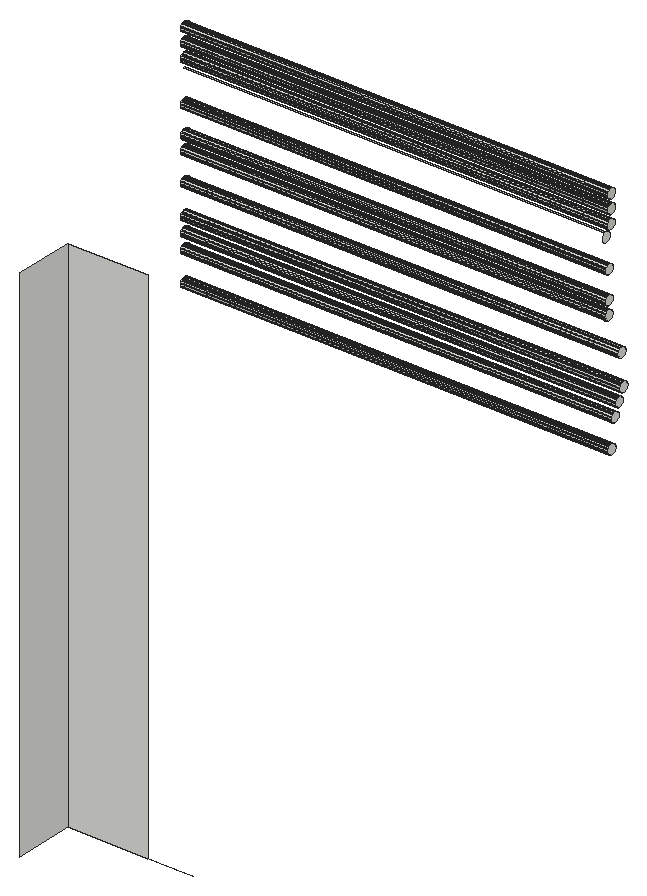
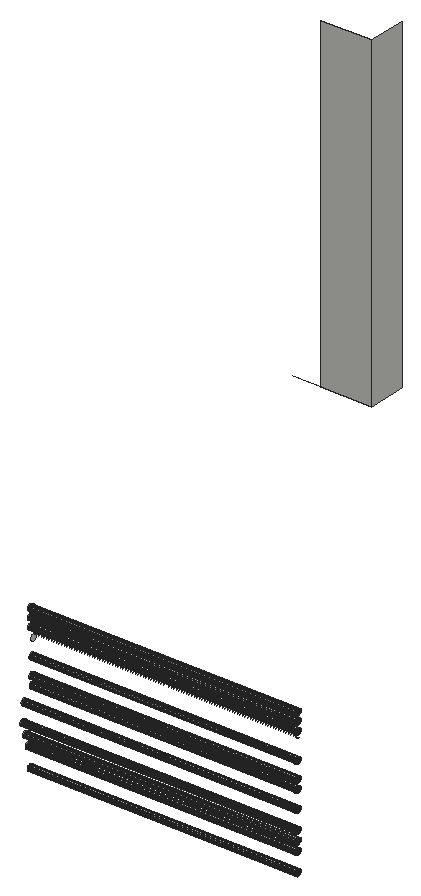
# SketchUp Ruby script. Lengths in inches.
U = 1.inch
M = Sketchup.active_model
def pt(a) = Geom::Point3d.new(a.map { |v| v * U })
def face(e, loops, mat)
  f = e.add_face(loops[0].map { |a| pt(a) })
  loops[1..].each { |l| e.add_face(l.map { |a| pt(a) }).erase! }
  f.material = f.back_material = mat if mat
  f
end
# faces: each face lists its corners as indices into pts; further lists are holes
def faces(e, pts, list, mat = nil) = list.each { |f| face(e, (f[0].is_a?(Array) ? f : [f]).map { |l| l.map { |i| pts[i] } }, mat) }
# xy, xz, yz: faces in a plane at the given z, y or x. An outline is a flat list of corners, or four numbers for a rectangle; further outlines are holes
def ring(l) = l.size == 4 ? [[l[0], l[1]], [l[2], l[1]], [l[2], l[3]], [l[0], l[3]]] : l.each_slice(2).to_a
def flat(e, list, mat, &to3) = list.each { |f| face(e, (f[0].is_a?(Array) ? f : [f]).map { |l| ring(l).map { |u, v| to3.(u, v) } }, mat) }
def xy(e, z, list, mat = nil) = flat(e, list, mat) { |x, y| [x, y, z] }
def xz(e, y, list, mat = nil) = flat(e, list, mat) { |x, z| [x, y, z] }
def yz(e, x, list, mat = nil) = flat(e, list, mat) { |y, z| [x, y, z] }
def lines(e, pts, list) = list.each { |a, b| e.add_line(pt(pts[a]), pt(pts[b])) }
# prism: a flat outline (further loops are holes) pulled along v
def prism(e, loops, v, mat = nil)
  f = face(e, loops, mat); d = Geom::Vector3d.new(v.map { |x| x * U })
  f.pushpull(f.normal.samedirection?(d) ? d.length : -d.length)
end
def box(e, o, s, mat = nil) = prism(e, [[o, [o[0] + s[0], o[1], o[2]], [o[0] + s[0], o[1] + s[1], o[2]], [o[0], o[1] + s[1], o[2]]]], [0, 0, s[2]], mat)
def at(x, y, z, deg = 0) = Geom::Transformation.translation(pt([x, y, z])) * Geom::Transformation.rotation(ORIGIN, Z_AXIS, deg.degrees)
def axes(o, x, y, z) = Geom::Transformation.new([*x, 0, *y, 0, *z, 0, *pt(o).to_a, 1])
def part(name) = M.definitions.add(name)
# library, detail: a bought-in or finely detailed component or shape, given as its bounding box
def library(name, o, s) = part(name).tap { |d| box(d.entities, o, s) }
def detail(e, o, s) = box(e.add_group.entities, o, s)
def put(e, d, t, mat = nil) = e.add_instance(d, t).tap { |i| i.material = mat if mat }
def group(e, t, mat = nil) = e.add_group.tap { |g| g.transformation = t; g.material = mat if mat }.entities
root = M.entities
M.materials.add("[Terrazzo Tile Light]").color = [219, 217, 210]
xz(root,74.42,[[587.04,144,603,248.36]])
yz(root,557.42,[[245.69,162.95,245.94,162.98,246.16,163.08,246.36,163.23,246.5,163.42,246.6,163.65,246.63,163.89,246.6,164.13,246.5,164.36,246.36,164.55,246.16,164.7,245.94,164.79,245.69,164.83,245.45,164.79,245.22,164.7,245.03,164.55,244.88,164.36,244.79,164.13,244.75,163.89,244.79,163.65,244.88,163.42,245.03,163.23,245.22,163.08,245.45,162.98]])
yz(root,557.98,[[245.69,149.2,245.94,149.23,246.16,149.33,246.36,149.48,246.5,149.67,246.6,149.9,246.63,150.14,246.6,150.38,246.5,150.61,246.36,150.8,246.16,150.95,245.94,151.04,245.69,151.08,245.45,151.04,245.22,150.95,245.03,150.8,244.88,150.61,244.79,150.38,244.75,150.14,244.79,149.9,244.88,149.67,245.03,149.48,245.22,149.33,245.45,149.23]])
yz(root,558.04,[[245.69,151.95,245.94,151.98,246.16,152.08,246.36,152.23,246.5,152.42,246.6,152.65,246.63,152.89,246.6,153.13,246.5,153.36,246.36,153.55,246.16,153.7,245.94,153.79,245.69,153.83,245.45,153.79,245.22,153.7,245.03,153.55,244.88,153.36,244.79,153.13,244.75,152.89,244.79,152.65,244.88,152.42,245.03,152.23,245.22,152.08,245.45,151.98],[245.69,157.45,245.94,157.48,246.16,157.58,246.36,157.73,246.5,157.92,246.6,158.15,246.63,158.39,246.6,158.63,246.5,158.86,246.36,159.05,246.16,159.2,245.94,159.29,245.69,159.33,245.45,159.29,245.22,159.2,245.03,159.05,244.88,158.86,244.79,158.63,244.75,158.39,244.79,158.15,244.88,157.92,245.03,157.73,245.22,157.58,245.45,157.48]])
yz(root,558.42,[[245.69,165.7,245.94,165.73,246.16,165.83,246.36,165.98,246.5,166.17,246.6,166.4,246.63,166.64,246.6,166.88,246.5,167.11,246.36,167.3,246.16,167.45,245.94,167.54,245.69,167.58,245.45,167.54,245.22,167.45,245.03,167.3,244.88,167.11,244.79,166.88,244.75,166.64,244.79,166.4,244.88,166.17,245.03,165.98,245.22,165.83,245.45,165.73]],"[Terrazzo Tile Light]")
yz(root,558.48,[[245.69,168.45,245.94,168.48,246.16,168.58,246.36,168.73,246.5,168.92,246.6,169.15,246.63,169.39,246.6,169.63,246.5,169.86,246.36,170.05,246.16,170.2,245.94,170.29,245.69,170.33,245.45,170.29,245.22,170.2,245.03,170.05,244.88,169.86,244.79,169.63,244.75,169.39,244.79,169.15,244.88,168.92,245.03,168.73,245.22,168.58,245.45,168.48],[245.69,171.2,245.94,171.23,246.16,171.33,246.36,171.48,246.5,171.67,246.6,171.9,246.63,172.14,246.6,172.38,246.5,172.61,246.36,172.8,246.16,172.95,245.94,173.04,245.69,173.08,245.45,173.04,245.22,172.95,245.03,172.8,244.88,172.61,244.79,172.38,244.75,172.14,244.79,171.9,244.88,171.67,245.03,171.48,245.22,171.33,245.45,171.23]],"[Terrazzo Tile Light]")
yz(root,558.54,[[245.69,125.45,245.94,125.48,246.16,125.58,246.36,125.73,246.5,125.92,246.6,126.15,246.63,126.39,246.6,126.63,246.5,126.86,246.36,127.05,246.16,127.2,245.94,127.29,245.69,127.33,245.45,127.29,245.22,127.2,245.03,127.05,244.88,126.86,244.79,126.63,244.75,126.39,244.79,126.15,244.88,125.92,245.03,125.73,245.22,125.58,245.45,125.48]])
yz(root,559.23,[[245.69,131.45,245.94,131.48,246.16,131.58,246.36,131.73,246.5,131.92,246.6,132.15,246.63,132.39,246.6,132.63,246.5,132.86,246.36,133.05,246.16,133.2,245.94,133.29,245.69,133.33,245.45,133.29,245.22,133.2,245.03,133.05,244.88,132.86,244.79,132.63,244.75,132.39,244.79,132.15,244.88,131.92,245.03,131.73,245.22,131.58,245.45,131.48]])
yz(root,560.04,[[245.69,134.45,245.94,134.48,246.16,134.58,246.36,134.73,246.5,134.92,246.6,135.15,246.63,135.39,246.6,135.63,246.5,135.86,246.36,136.05,246.16,136.2,245.94,136.29,245.69,136.33,245.45,136.29,245.22,136.2,245.03,136.05,244.88,135.86,244.79,135.63,244.75,135.39,244.79,135.15,244.88,134.92,245.03,134.73,245.22,134.58,245.45,134.48]])
yz(root,560.54,[[245.69,143.45,245.94,143.48,246.16,143.58,246.36,143.73,246.5,143.92,246.6,144.15,246.63,144.39,246.6,144.63,246.5,144.86,246.36,145.05,246.16,145.2,245.94,145.29,245.69,145.33,245.45,145.29,245.22,145.2,245.03,145.05,244.88,144.86,244.79,144.63,244.75,144.39,244.79,144.15,244.88,143.92,245.03,143.73,245.22,143.58,245.45,143.48]])
yz(root,560.92,[[245.69,137.45,245.94,137.48,246.16,137.58,246.36,137.73,246.5,137.92,246.6,138.15,246.63,138.39,246.6,138.63,246.5,138.86,246.36,139.05,246.16,139.2,245.94,139.29,245.69,139.33,245.45,139.29,245.22,139.2,245.03,139.05,244.88,138.86,244.79,138.63,244.75,138.39,244.79,138.15,244.88,137.92,245.03,137.73,245.22,137.58,245.45,137.48]])
yz(root,587.04,[[62.42,144,74.42,248.36]])
p = [[473.23,245.22,125.58],[473.23,245.45,125.48],[558.54,245.45,125.48],[558.54,245.22,125.58],[473.23,245.69,125.45],[558.54,245.69,125.45],
  [473.23,245.94,125.48],[558.54,245.94,125.48],[473.23,246.16,125.58],[558.54,246.16,125.58],[473.23,245.03,125.73],[558.54,245.03,125.73],
  [473.23,246.36,125.73],[558.54,246.36,125.73],[473.23,244.88,125.92],[558.54,244.88,125.92],[473.23,246.5,125.92],[558.54,246.5,125.92],
  [473.23,244.79,126.15],[558.54,244.79,126.15],[473.23,246.6,126.15],[558.54,246.6,126.15],[473.23,244.75,126.39],[558.54,244.75,126.39],
  [473.23,246.63,126.39],[558.54,246.63,126.39],[473.23,244.79,126.63],[558.54,244.79,126.63],[473.23,246.6,126.63],[558.54,246.6,126.63],
  [473.23,244.88,126.86],[558.54,244.88,126.86],[473.23,246.5,126.86],[558.54,246.5,126.86],[473.23,245.03,127.05],[558.54,245.03,127.05],
  [473.23,246.36,127.05],[558.54,246.36,127.05],[473.23,245.22,127.2],[558.54,245.22,127.2],[473.23,246.16,127.2],[558.54,246.16,127.2],
  [473.23,245.45,127.29],[558.54,245.45,127.29],[473.23,245.94,127.29],[558.54,245.94,127.29],[473.23,245.69,127.33],[558.54,245.69,127.33],
  [473.23,245.22,131.58],[473.23,245.45,131.48],[559.23,245.45,131.48],[559.23,245.22,131.58],[473.23,245.69,131.45],[559.23,245.69,131.45],
  [473.23,245.94,131.48],[559.23,245.94,131.48],[473.23,246.16,131.58],[559.23,246.16,131.58],[473.23,245.03,131.73],[559.23,245.03,131.73],
  [473.23,246.36,131.73],[559.23,246.36,131.73],[473.23,244.88,131.92],[559.23,244.88,131.92],[473.23,246.5,131.92],[559.23,246.5,131.92],
  [473.23,244.79,132.15],[559.23,244.79,132.15],[473.23,246.6,132.15],[559.23,246.6,132.15],[473.23,244.75,132.39],[559.23,244.75,132.39],
  [473.23,246.63,132.39],[559.23,246.63,132.39],[473.23,244.79,132.63],[559.23,244.79,132.63],[473.23,246.6,132.63],[559.23,246.6,132.63],
  [473.23,244.88,132.86],[559.23,244.88,132.86],[473.23,246.5,132.86],[559.23,246.5,132.86],[473.23,245.03,133.05],[559.23,245.03,133.05],
  [473.23,246.36,133.05],[559.23,246.36,133.05],[473.23,245.22,133.2],[559.23,245.22,133.2],[473.23,246.16,133.2],[559.23,246.16,133.2],
  [473.23,245.45,133.29],[559.23,245.45,133.29],[473.23,245.94,133.29],[559.23,245.94,133.29],[473.23,245.69,133.33],[559.23,245.69,133.33],
  [473.23,245.22,134.58],[473.23,245.45,134.48],[560.04,245.45,134.48],[560.04,245.22,134.58],[473.23,245.69,134.45],[560.04,245.69,134.45],
  [473.23,245.94,134.48],[560.04,245.94,134.48],[473.23,246.16,134.58],[560.04,246.16,134.58],[473.23,245.03,134.73],[560.04,245.03,134.73],
  [473.23,246.36,134.73],[560.04,246.36,134.73],[473.23,244.88,134.92],[560.04,244.88,134.92],[473.23,246.5,134.92],[560.04,246.5,134.92],
  [473.23,244.79,135.15],[560.04,244.79,135.15],[473.23,246.6,135.15],[560.04,246.6,135.15],[473.23,244.75,135.39],[560.04,244.75,135.39],
  [473.23,246.63,135.39],[560.04,246.63,135.39],[473.23,244.79,135.63],[560.04,244.79,135.63],[473.23,246.6,135.63],[560.04,246.6,135.63],
  [473.23,244.88,135.86],[560.04,244.88,135.86],[473.23,246.5,135.86],[560.04,246.5,135.86],[473.23,245.03,136.05],[560.04,245.03,136.05],
  [473.23,246.36,136.05],[560.04,246.36,136.05],[473.23,245.22,136.2],[560.04,245.22,136.2],[473.23,246.16,136.2],[560.04,246.16,136.2],
  [473.23,245.45,136.29],[560.04,245.45,136.29],[473.23,245.94,136.29],[560.04,245.94,136.29],[473.23,245.69,136.33],[560.04,245.69,136.33],
  [473.23,245.22,137.58],[473.23,245.45,137.48],[560.92,245.45,137.48],[560.92,245.22,137.58],[473.23,245.69,137.45],[560.92,245.69,137.45],
  [473.23,245.94,137.48],[560.92,245.94,137.48],[473.23,246.16,137.58],[560.92,246.16,137.58],[473.23,245.03,137.73],[560.92,245.03,137.73],
  [473.23,246.36,137.73],[560.92,246.36,137.73],[473.23,244.88,137.92],[560.92,244.88,137.92],[473.23,246.5,137.92],[560.92,246.5,137.92],
  [473.23,244.79,138.15],[560.92,244.79,138.15],[473.23,246.6,138.15],[560.92,246.6,138.15],[473.23,244.75,138.39],[560.92,244.75,138.39],
  [473.23,246.63,138.39],[560.92,246.63,138.39],[473.23,244.79,138.63],[560.92,244.79,138.63],[473.23,246.6,138.63],[560.92,246.6,138.63],
  [473.23,244.88,138.86],[560.92,244.88,138.86],[473.23,246.5,138.86],[560.92,246.5,138.86],[473.23,245.03,139.05],[560.92,245.03,139.05],
  [473.23,246.36,139.05],[560.92,246.36,139.05],[473.23,245.22,139.2],[560.92,245.22,139.2],[473.23,246.16,139.2],[560.92,246.16,139.2],
  [473.23,245.45,139.29],[560.92,245.45,139.29],[473.23,245.94,139.29],[560.92,245.94,139.29],[473.23,245.69,139.33],[560.92,245.69,139.33],
  [473.23,245.22,143.58],[473.23,245.45,143.48],[560.54,245.45,143.48],[560.54,245.22,143.58],[473.23,245.69,143.45],[560.54,245.69,143.45],
  [473.23,245.94,143.48],[560.54,245.94,143.48],[473.23,246.16,143.58],[560.54,246.16,143.58],[473.23,245.03,143.73],[560.54,245.03,143.73],
  [473.23,246.36,143.73],[560.54,246.36,143.73],[473.23,244.88,143.92],[560.54,244.88,143.92],[473.23,246.5,143.92],[560.54,246.5,143.92],
  [473.23,244.79,144.15],[560.54,244.79,144.15],[473.23,246.6,144.15],[560.54,246.6,144.15],[473.23,244.75,144.39],[560.54,244.75,144.39],
  [473.23,246.63,144.39],[560.54,246.63,144.39],[473.23,244.79,144.63],[560.54,244.79,144.63],[473.23,246.6,144.63],[560.54,246.6,144.63],
  [473.23,244.88,144.86],[560.54,244.88,144.86],[473.23,246.5,144.86],[560.54,246.5,144.86],[473.23,245.03,145.05],[560.54,245.03,145.05],
  [473.23,246.36,145.05],[560.54,246.36,145.05],[473.23,245.22,145.2],[560.54,245.22,145.2],[473.23,246.16,145.2],[560.54,246.16,145.2],
  [473.23,245.45,145.29],[560.54,245.45,145.29],[473.23,245.94,145.29],[560.54,245.94,145.29],[473.23,245.69,145.33],[560.54,245.69,145.33],
  [473.23,245.22,149.33],[473.23,245.45,149.23],[557.98,245.45,149.23],[557.98,245.22,149.33],[473.23,245.69,149.2],[557.98,245.69,149.2],
  [473.23,245.94,149.23],[557.98,245.94,149.23],[473.23,246.16,149.33],[557.98,246.16,149.33],[473.23,245.03,149.48],[557.98,245.03,149.48],
  [473.23,246.36,149.48],[557.98,246.36,149.48],[473.23,244.88,149.67],[557.98,244.88,149.67],[473.23,246.5,149.67],[557.98,246.5,149.67],
  [473.23,244.79,149.9],[557.98,244.79,149.9],[473.23,246.6,149.9],[557.98,246.6,149.9],[473.23,244.75,150.14],[557.98,244.75,150.14],
  [473.23,246.63,150.14],[557.98,246.63,150.14],[473.23,244.79,150.38],[557.98,244.79,150.38],[473.23,246.6,150.38],[557.98,246.6,150.38],
  [473.23,244.88,150.61],[557.98,244.88,150.61],[473.23,246.5,150.61],[557.98,246.5,150.61],[473.23,245.03,150.8],[557.98,245.03,150.8],
  [473.23,246.36,150.8],[557.98,246.36,150.8],[473.23,245.22,150.95],[557.98,245.22,150.95],[473.23,246.16,150.95],[557.98,246.16,150.95],
  [473.23,245.45,151.04],[557.98,245.45,151.04],[473.23,245.69,151.08],[557.98,245.69,151.08],[473.23,245.94,151.04],[557.98,245.94,151.04],
  [473.23,245.22,152.08],[473.23,245.45,151.98],[558.04,245.45,151.98],[558.04,245.22,152.08],[473.23,245.69,151.95],[558.04,245.69,151.95],
  [473.23,245.94,151.98],[558.04,245.94,151.98],[473.23,246.16,152.08],[558.04,246.16,152.08],[473.23,245.03,152.23],[558.04,245.03,152.23],
  [473.23,246.36,152.23],[558.04,246.36,152.23],[473.23,244.88,152.42],[558.04,244.88,152.42],[473.23,246.5,152.42],[558.04,246.5,152.42],
  [473.23,244.79,152.65],[558.04,244.79,152.65],[473.23,246.6,152.65],[558.04,246.6,152.65],[473.23,244.75,152.89],[558.04,244.75,152.89],
  [473.23,246.63,152.89],[558.04,246.63,152.89],[473.23,244.79,153.13],[558.04,244.79,153.13],[473.23,246.6,153.13],[558.04,246.6,153.13],
  [473.23,244.88,153.36],[558.04,244.88,153.36],[473.23,246.5,153.36],[558.04,246.5,153.36],[473.23,245.03,153.55],[558.04,245.03,153.55],
  [473.23,246.36,153.55],[558.04,246.36,153.55],[473.23,245.22,153.7],[558.04,245.22,153.7],[473.23,246.16,153.7],[558.04,246.16,153.7],
  [473.23,245.45,153.79],[558.04,245.45,153.79],[473.23,245.94,153.79],[558.04,245.94,153.79],[473.23,245.69,153.83],[558.04,245.69,153.83],
  [473.23,245.22,157.58],[473.23,245.45,157.48],[558.04,245.45,157.48],[558.04,245.22,157.58],[473.23,245.69,157.45],[558.04,245.69,157.45],
  [473.23,245.94,157.48],[558.04,245.94,157.48],[473.23,246.16,157.58],[558.04,246.16,157.58],[473.23,245.03,157.73],[558.04,245.03,157.73],
  [473.23,246.36,157.73],[558.04,246.36,157.73],[473.23,244.88,157.92],[558.04,244.88,157.92],[473.23,246.5,157.92],[558.04,246.5,157.92],
  [473.23,244.79,158.15],[558.04,244.79,158.15],[473.23,246.6,158.15],[558.04,246.6,158.15],[473.23,244.75,158.39],[558.04,244.75,158.39],
  [473.23,246.63,158.39],[558.04,246.63,158.39],[473.23,244.79,158.63],[558.04,244.79,158.63],[473.23,246.6,158.63],[558.04,246.6,158.63],
  [473.23,244.88,158.86],[558.04,244.88,158.86],[473.23,246.5,158.86],[558.04,246.5,158.86],[473.23,245.03,159.05],[558.04,245.03,159.05],
  [473.23,246.36,159.05],[558.04,246.36,159.05],[473.23,245.22,159.2],[558.04,245.22,159.2],[473.23,246.16,159.2],[558.04,246.16,159.2],
  [473.23,245.45,159.29],[558.04,245.45,159.29],[473.23,245.94,159.29],[558.04,245.94,159.29],[473.23,245.69,159.33],[558.04,245.69,159.33],
  [473.23,245.69,164.83],[473.23,245.45,164.79],[557.42,245.45,164.79],[557.42,245.69,164.83],[473.23,245.22,165.83],[473.23,245.45,165.73],
  [558.42,245.45,165.73],[558.42,245.22,165.83],[473.23,245.69,165.7],[558.42,245.69,165.7],[473.23,245.94,165.73],[558.42,245.94,165.73],
  [473.23,246.16,165.83],[558.42,246.16,165.83],[473.23,245.03,165.98],[558.42,245.03,165.98],[473.23,246.36,165.98],[558.42,246.36,165.98],
  [473.23,244.88,166.17],[558.42,244.88,166.17],[473.23,246.5,166.17],[558.42,246.5,166.17],[473.23,244.79,166.4],[558.42,244.79,166.4],
  [473.23,246.6,166.4],[558.42,246.6,166.4],[473.23,244.75,166.64],[558.42,244.75,166.64],[473.23,246.63,166.64],[558.42,246.63,166.64],
  [473.23,244.79,166.88],[558.42,244.79,166.88],[473.23,246.6,166.88],[558.42,246.6,166.88],[473.23,244.88,167.11],[558.42,244.88,167.11],
  [473.23,246.5,167.11],[558.42,246.5,167.11],[473.23,245.03,167.3],[558.42,245.03,167.3],[473.23,246.36,167.3],[558.42,246.36,167.3],
  [473.23,245.22,167.45],[558.42,245.22,167.45],[473.23,246.16,167.45],[558.42,246.16,167.45],[473.23,245.45,167.54],[558.42,245.45,167.54],
  [473.23,245.69,167.58],[558.42,245.69,167.58],[473.23,245.94,167.54],[558.42,245.94,167.54],[473.23,245.22,168.58],[473.23,245.45,168.48],
  [558.48,245.45,168.48],[558.48,245.22,168.58],[473.23,245.69,168.45],[558.48,245.69,168.45],[473.23,245.94,168.48],[558.48,245.94,168.48],
  [473.23,246.16,168.58],[558.48,246.16,168.58],[473.23,245.03,168.73],[558.48,245.03,168.73],[473.23,246.36,168.73],[558.48,246.36,168.73],
  [473.23,244.88,168.92],[558.48,244.88,168.92],[473.23,246.5,168.92],[558.48,246.5,168.92],[473.23,244.79,169.15],[558.48,244.79,169.15],
  [473.23,246.6,169.15],[558.48,246.6,169.15],[473.23,244.75,169.39],[558.48,244.75,169.39],[473.23,246.63,169.39],[558.48,246.63,169.39],
  [473.23,244.79,169.63],[558.48,244.79,169.63],[473.23,246.6,169.63],[558.48,246.6,169.63],[473.23,244.88,169.86],[558.48,244.88,169.86],
  [473.23,246.5,169.86],[558.48,246.5,169.86],[473.23,245.03,170.05],[558.48,245.03,170.05],[473.23,246.36,170.05],[558.48,246.36,170.05],
  [473.23,245.22,170.2],[558.48,245.22,170.2],[473.23,246.16,170.2],[558.48,246.16,170.2],[473.23,245.45,170.29],[558.48,245.45,170.29],
  [473.23,245.94,170.29],[558.48,245.94,170.29],[473.23,245.69,170.33],[558.48,245.69,170.33],[473.23,245.22,171.33],[473.23,245.45,171.23],
  [558.48,245.45,171.23],[558.48,245.22,171.33],[473.23,245.69,171.2],[558.48,245.69,171.2],[473.23,245.94,171.23],[558.48,245.94,171.23],
  [473.23,246.16,171.33],[558.48,246.16,171.33],[473.23,245.03,171.48],[558.48,245.03,171.48],[473.23,246.36,171.48],[558.48,246.36,171.48],
  [473.23,244.88,171.67],[558.48,244.88,171.67],[473.23,246.5,171.67],[558.48,246.5,171.67],[473.23,244.79,171.9],[558.48,244.79,171.9],
  [473.23,246.6,171.9],[558.48,246.6,171.9],[473.23,244.75,172.14],[558.48,244.75,172.14],[473.23,246.63,172.14],[558.48,246.63,172.14],
  [473.23,244.79,172.38],[558.48,244.79,172.38],[473.23,246.6,172.38],[558.48,246.6,172.38],[473.23,244.88,172.61],[558.48,244.88,172.61],
  [473.23,246.5,172.61],[558.48,246.5,172.61],[473.23,245.03,172.8],[558.48,245.03,172.8],[473.23,246.36,172.8],[558.48,246.36,172.8],
  [473.23,245.22,172.95],[558.48,245.22,172.95],[473.23,246.16,172.95],[558.48,246.16,172.95],[473.23,245.45,173.04],[558.48,245.45,173.04],
  [473.23,245.69,173.08],[558.48,245.69,173.08],[473.23,245.94,173.04],[558.48,245.94,173.04],[603,74.42,144],[612,74.42,144]]
faces(root,p,[[0,1,2,3],[1,4,5,2],[4,6,7,5],[6,8,9,7],[10,0,3,11],[8,12,13,9],[14,10,11,15],[12,16,17,13],
  [18,14,15,19],[16,20,21,17],[22,18,19,23],[20,24,25,21],[26,22,23,27],[24,28,29,25],[30,26,27,31],[28,32,33,29],
  [34,30,31,35],[32,36,37,33],[38,34,35,39],[36,40,41,37],[42,38,39,43],[40,44,45,41],[46,42,43,47],[44,46,47,45],
  [48,49,50,51],[49,52,53,50],[52,54,55,53],[54,56,57,55],[58,48,51,59],[56,60,61,57],[62,58,59,63],[60,64,65,61],
  [66,62,63,67],[64,68,69,65],[70,66,67,71],[68,72,73,69],[74,70,71,75],[72,76,77,73],[78,74,75,79],[76,80,81,77],
  [82,78,79,83],[80,84,85,81],[86,82,83,87],[84,88,89,85],[90,86,87,91],[88,92,93,89],[94,90,91,95],[92,94,95,93],
  [96,97,98,99],[97,100,101,98],[100,102,103,101],[102,104,105,103],[106,96,99,107],[104,108,109,105],[110,106,107,111],[108,112,113,109],
  [114,110,111,115],[112,116,117,113],[118,114,115,119],[116,120,121,117],[122,118,119,123],[120,124,125,121],[126,122,123,127],[124,128,129,125],
  [130,126,127,131],[128,132,133,129],[134,130,131,135],[132,136,137,133],[138,134,135,139],[136,140,141,137],[142,138,139,143],[140,142,143,141],
  [144,145,146,147],[145,148,149,146],[148,150,151,149],[150,152,153,151],[154,144,147,155],[152,156,157,153],[158,154,155,159],[156,160,161,157],
  [162,158,159,163],[160,164,165,161],[166,162,163,167],[164,168,169,165],[170,166,167,171],[168,172,173,169],[174,170,171,175],[172,176,177,173],
  [178,174,175,179],[176,180,181,177],[182,178,179,183],[180,184,185,181],[186,182,183,187],[184,188,189,185],[190,186,187,191],[188,190,191,189],
  [192,193,194,195],[193,196,197,194],[196,198,199,197],[198,200,201,199],[202,192,195,203],[200,204,205,201],[206,202,203,207],[204,208,209,205],
  [210,206,207,211],[208,212,213,209],[214,210,211,215],[212,216,217,213],[218,214,215,219],[216,220,221,217],[222,218,219,223],[220,224,225,221],
  [226,222,223,227],[224,228,229,225],[230,226,227,231],[228,232,233,229],[234,230,231,235],[232,236,237,233],[238,234,235,239],[236,238,239,237],
  [240,241,242,243],[241,244,245,242],[244,246,247,245],[246,248,249,247],[250,240,243,251],[248,252,253,249],[254,250,251,255],[252,256,257,253],
  [258,254,255,259],[256,260,261,257],[262,258,259,263],[260,264,265,261],[266,262,263,267],[264,268,269,265],[270,266,267,271],[268,272,273,269],
  [274,270,271,275],[272,276,277,273],[278,274,275,279],[276,280,281,277],[282,278,279,283],[284,282,283,285],[286,284,285,287],[280,286,287,281],
  [288,289,290,291],[289,292,293,290],[292,294,295,293],[294,296,297,295],[298,288,291,299],[296,300,301,297],[302,298,299,303],[300,304,305,301],
  [306,302,303,307],[304,308,309,305],[310,306,307,311],[308,312,313,309],[314,310,311,315],[312,316,317,313],[318,314,315,319],[316,320,321,317],
  [322,318,319,323],[320,324,325,321],[326,322,323,327],[324,328,329,325],[330,326,327,331],[328,332,333,329],[334,330,331,335],[332,334,335,333],
  [336,337,338,339],[337,340,341,338],[340,342,343,341],[342,344,345,343],[346,336,339,347],[344,348,349,345],[350,346,347,351],[348,352,353,349],
  [354,350,351,355],[352,356,357,353],[358,354,355,359],[356,360,361,357],[362,358,359,363],[360,364,365,361],[366,362,363,367],[364,368,369,365],
  [370,366,367,371],[368,372,373,369],[374,370,371,375],[372,376,377,373],[378,374,375,379],[376,380,381,377],[382,378,379,383],[380,382,383,381],
  [384,385,386,387],[388,389,390,391],[389,392,393,390],[392,394,395,393],[394,396,397,395],[398,388,391,399],[396,400,401,397],[402,398,399,403],
  [400,404,405,401],[406,402,403,407],[404,408,409,405],[410,406,407,411],[408,412,413,409],[414,410,411,415],[412,416,417,413],[418,414,415,419],
  [416,420,421,417],[422,418,419,423],[420,424,425,421],[426,422,423,427],[424,428,429,425],[430,426,427,431],[432,430,431,433],[434,432,433,435],
  [428,434,435,429],[436,437,438,439],[437,440,441,438],[440,442,443,441],[442,444,445,443],[446,436,439,447],[444,448,449,445],[450,446,447,451],
  [448,452,453,449],[454,450,451,455],[452,456,457,453],[458,454,455,459],[456,460,461,457],[462,458,459,463],[460,464,465,461],[466,462,463,467],
  [464,468,469,465],[470,466,467,471],[468,472,473,469],[474,470,471,475],[472,476,477,473],[478,474,475,479],[476,480,481,477],[482,478,479,483],
  [480,482,483,481],[484,485,486,487],[485,488,489,486],[488,490,491,489],[490,492,493,491],[494,484,487,495],[492,496,497,493],[498,494,495,499],
  [496,500,501,497],[502,498,499,503],[500,504,505,501],[506,502,503,507],[504,508,509,505],[510,506,507,511],[508,512,513,509],[514,510,511,515],
  [512,516,517,513],[518,514,515,519],[516,520,521,517],[522,518,519,523],[520,524,525,521],[526,522,523,527],[528,526,527,529],[530,528,529,531],
  [524,530,531,525]],"[Terrazzo Tile Light]")
lines(root,p,[[532,533]])
